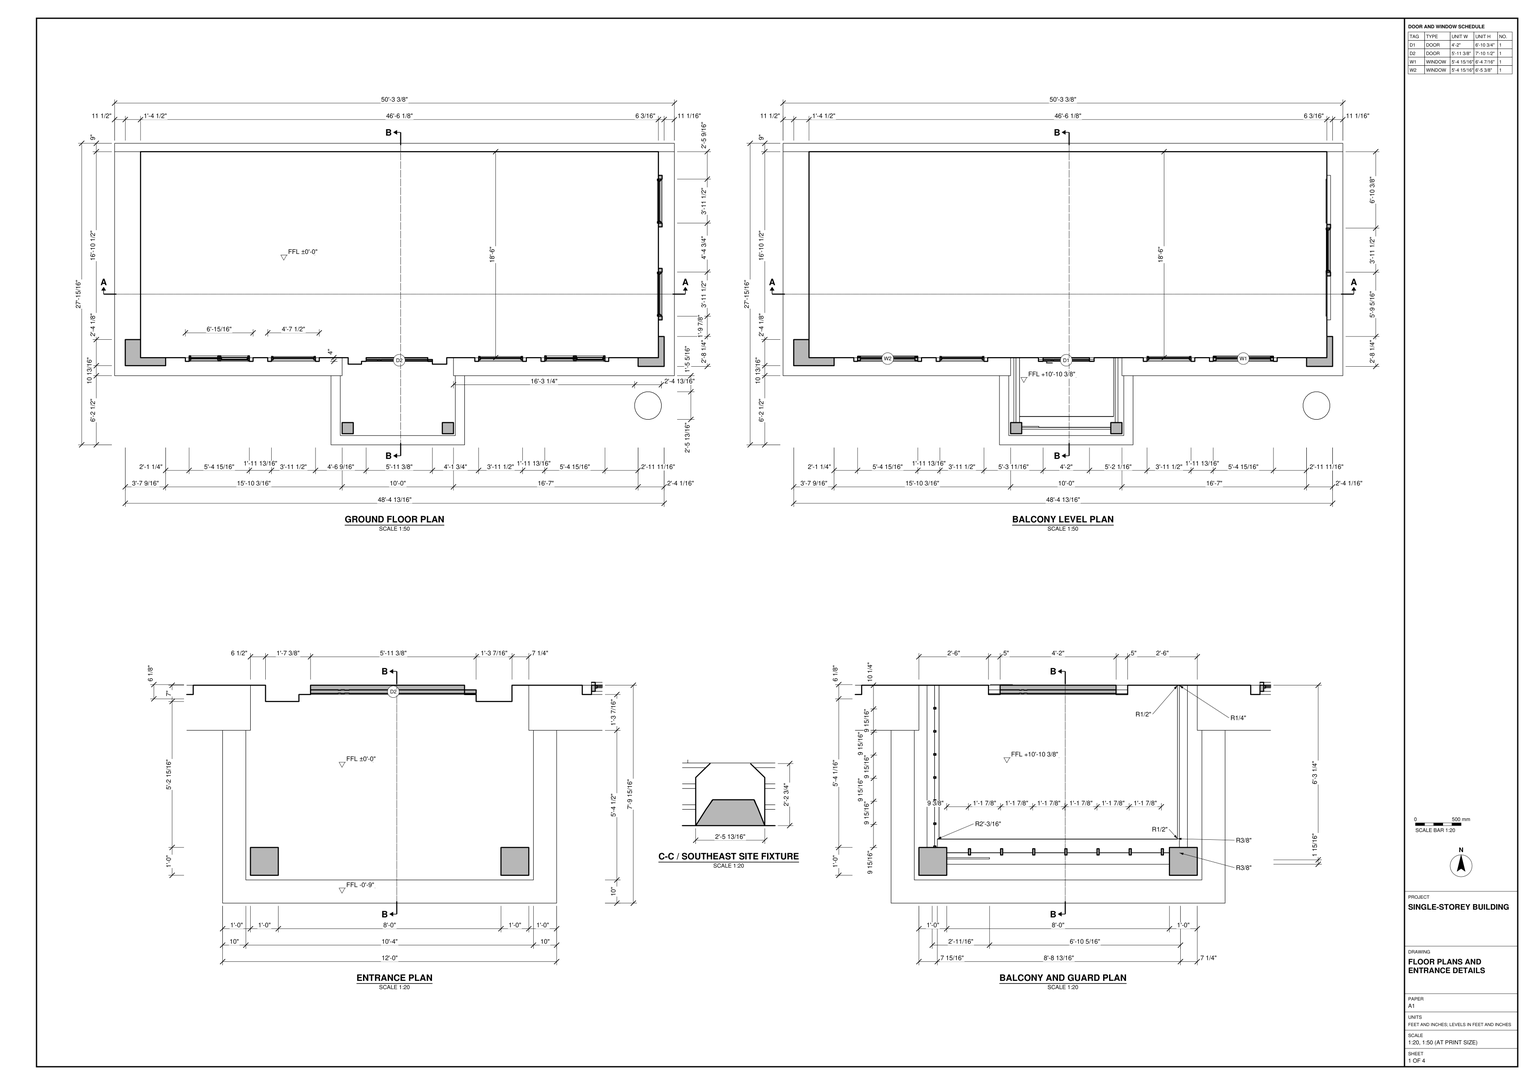
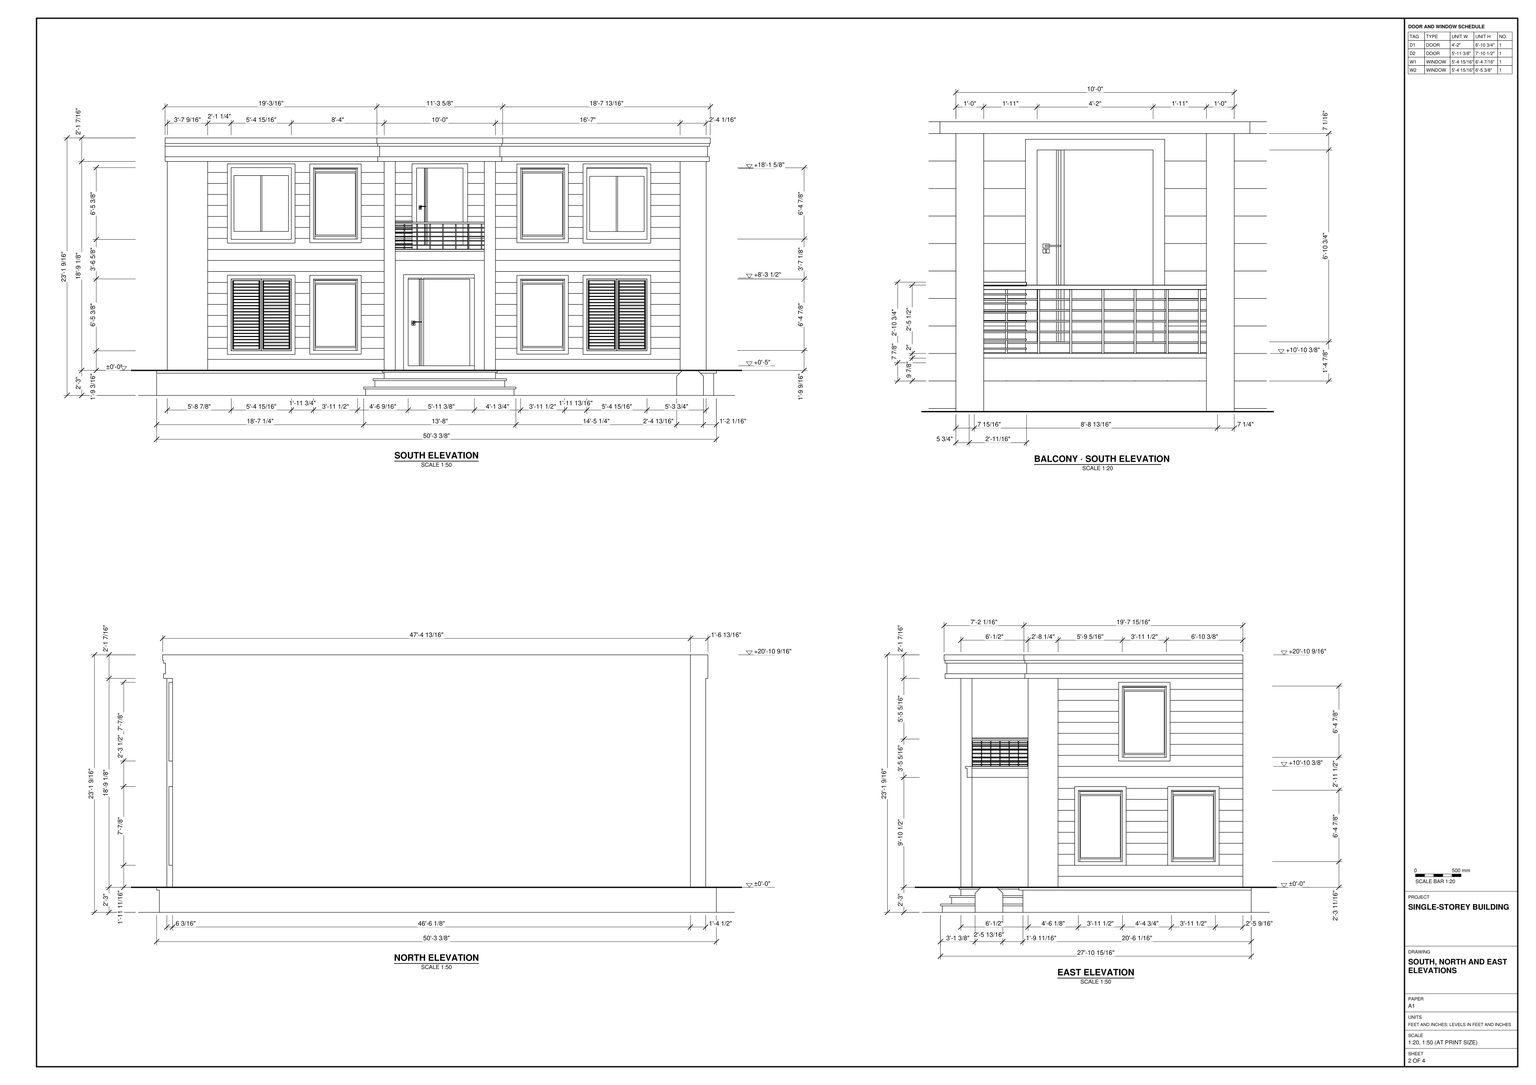
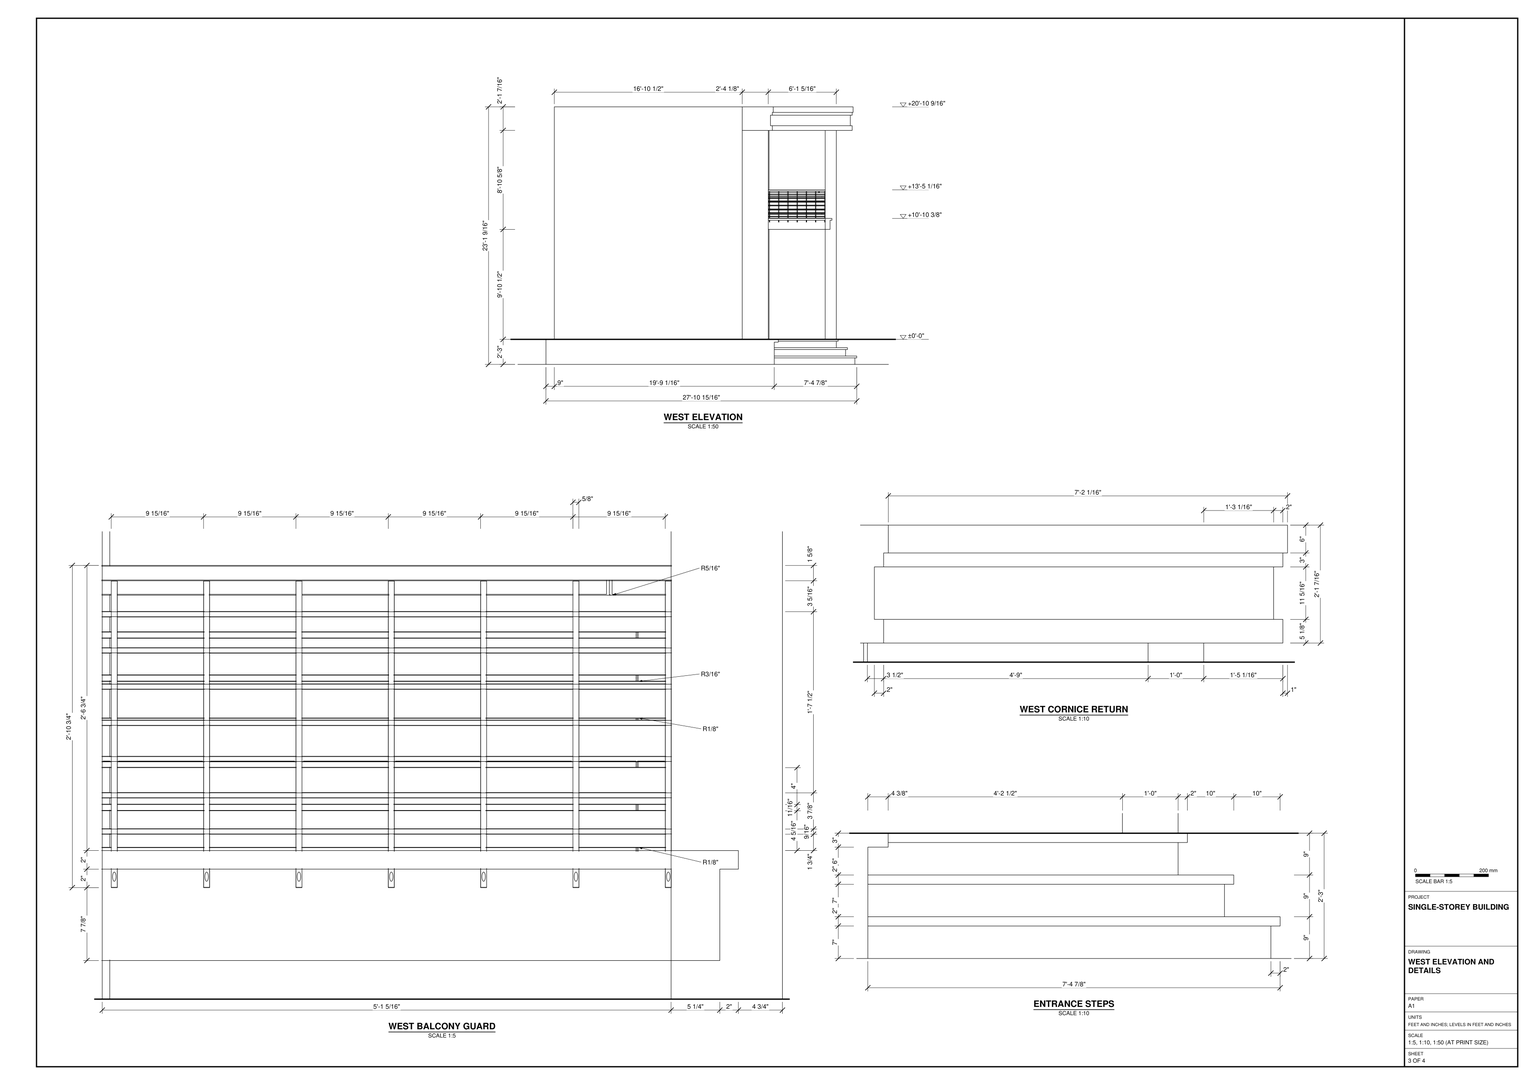
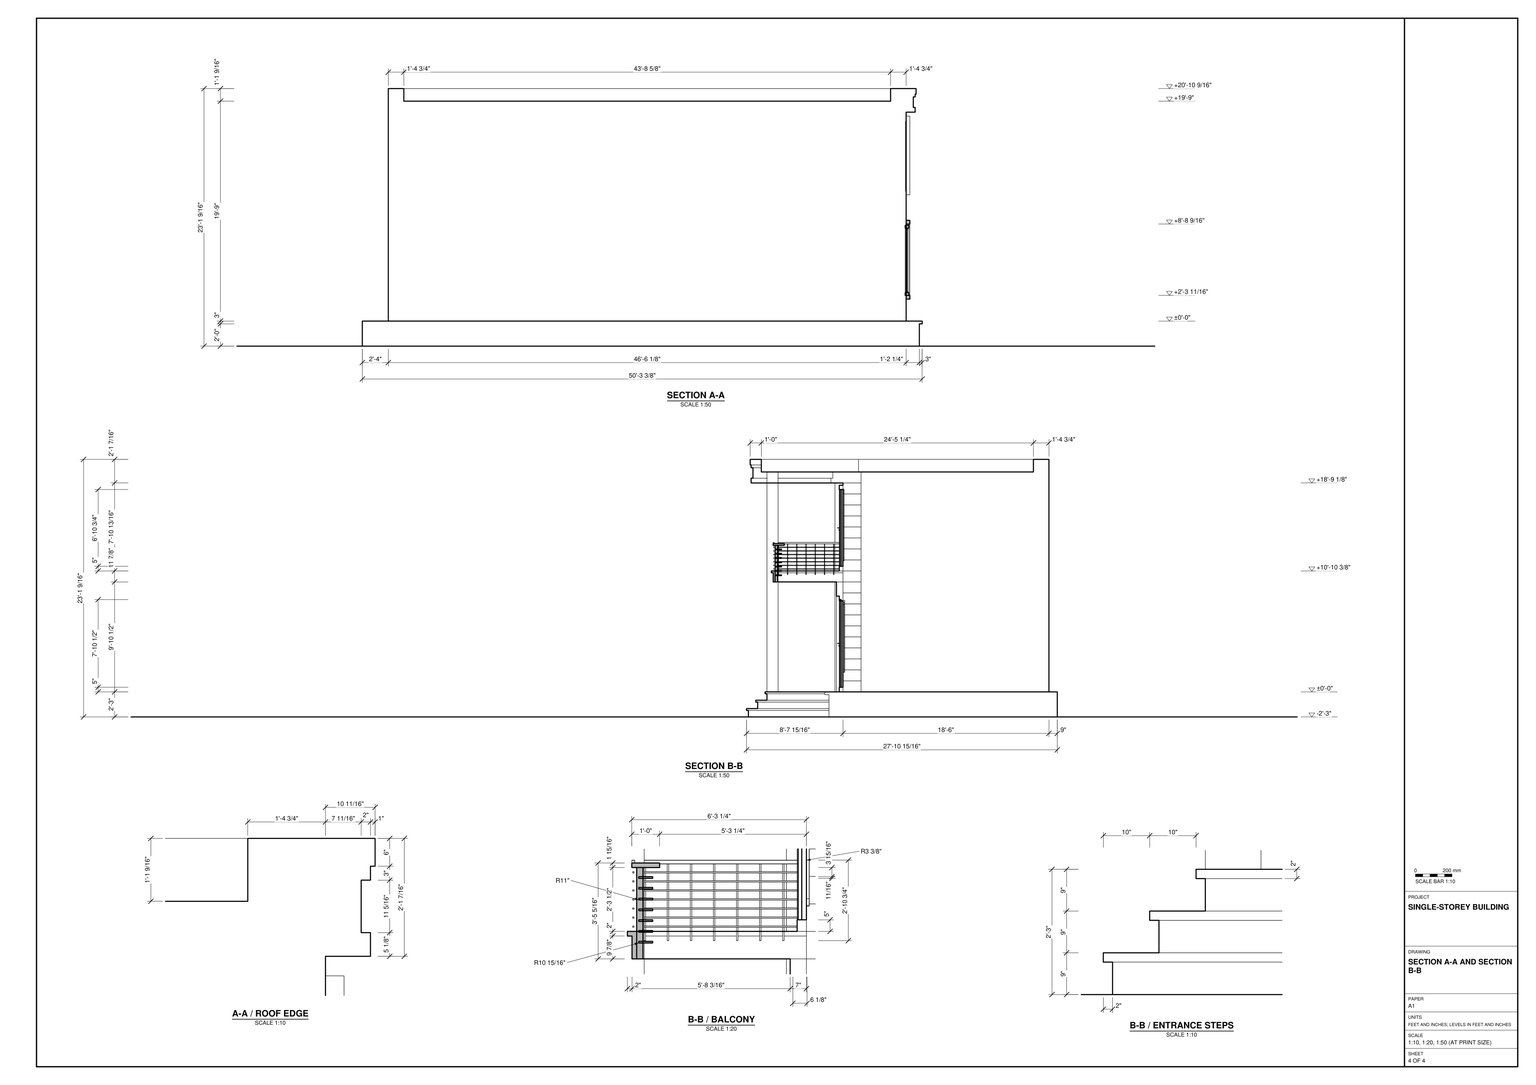
Build the single-storey building and its site in SketchUp using task_files/diagram_01.pdf. Work in feet and inches. The complete model, including the site, measures 82'-5 5/16" along X, 104'-8 7/8" along Y and 23'-1 9/16" along Z. Use ±0'-0" as the ground-floor level. Use the dimensioned plans, rather than the site extents, to set out the building footprint.

Model the floor slab, exterior walls at their drawn thicknesses, and roof with its stepped cornice. On the south face, build the entrance steps and landing beneath the projecting balcony. Align the balcony door over the entrance door, place the square supports at the outer corners, and carry the balcony guard across the front and along the sides. Follow the elevations for the window frames, louvred units and horizontal wall courses, noting how the east window arrangement differs from the south frontage. Include the site fixture shown southeast of the building.

Keep shell elements such as walls, slabs and roof, and any furniture or joinery pieces shown, in separate groups or components. Use components for repeated parts. Decor and loose items may be any suitable library components. Save one SketchUp model as output_files/single_storey_building_with_entrance_steps_and_balcony.skp.

# SketchUp Ruby script. Lengths in inches.
U = 1.inch
M = Sketchup.active_model
def pt(a) = Geom::Point3d.new(a.map { |v| v * U })
def face(e, loops, mat)
  f = e.add_face(loops[0].map { |a| pt(a) })
  loops[1..].each { |l| e.add_face(l.map { |a| pt(a) }).erase! }
  f.material = f.back_material = mat if mat
  f
end
# faces: each face lists its corners as indices into pts; further lists are holes
def faces(e, pts, list, mat = nil) = list.each { |f| face(e, (f[0].is_a?(Array) ? f : [f]).map { |l| l.map { |i| pts[i] } }, mat) }
# xy, xz, yz: faces in a plane at the given z, y or x. An outline is a flat list of corners, or four numbers for a rectangle; further outlines are holes
def ring(l) = l.size == 4 ? [[l[0], l[1]], [l[2], l[1]], [l[2], l[3]], [l[0], l[3]]] : l.each_slice(2).to_a
def flat(e, list, mat, &to3) = list.each { |f| face(e, (f[0].is_a?(Array) ? f : [f]).map { |l| ring(l).map { |u, v| to3.(u, v) } }, mat) }
def xy(e, z, list, mat = nil) = flat(e, list, mat) { |x, y| [x, y, z] }
def xz(e, y, list, mat = nil) = flat(e, list, mat) { |x, z| [x, y, z] }
def yz(e, x, list, mat = nil) = flat(e, list, mat) { |y, z| [x, y, z] }
def lines(e, pts, list) = list.each { |a, b| e.add_line(pt(pts[a]), pt(pts[b])) }
# prism: a flat outline (further loops are holes) pulled along v
def prism(e, loops, v, mat = nil)
  f = face(e, loops, mat); d = Geom::Vector3d.new(v.map { |x| x * U })
  f.pushpull(f.normal.samedirection?(d) ? d.length : -d.length)
end
def box(e, o, s, mat = nil) = prism(e, [[o, [o[0] + s[0], o[1], o[2]], [o[0] + s[0], o[1] + s[1], o[2]], [o[0], o[1] + s[1], o[2]]]], [0, 0, s[2]], mat)
def at(x, y, z, deg = 0) = Geom::Transformation.translation(pt([x, y, z])) * Geom::Transformation.rotation(ORIGIN, Z_AXIS, deg.degrees)
def axes(o, x, y, z) = Geom::Transformation.new([*x, 0, *y, 0, *z, 0, *pt(o).to_a, 1])
def part(name) = M.definitions.add(name)
# library, detail: a bought-in or finely detailed component or shape, given as its bounding box
def library(name, o, s) = part(name).tap { |d| box(d.entities, o, s) }
def detail(e, o, s) = box(e.add_group.entities, o, s)
def put(e, d, t, mat = nil) = e.add_instance(d, t).tap { |i| i.material = mat if mat }
def group(e, t, mat = nil) = e.add_group.tap { |g| g.transformation = t; g.material = mat if mat }.entities
root = M.entities
M.materials.add("GATE RAILINGS").color = [40, 40, 40]
M.materials.add("[0049_Beige]").color = [245, 245, 220]
M.materials.add("[0135_DarkGray]").color = [81, 81, 81]
M.materials.add("[Color_009]").color = [0, 0, 0]
M.materials.add("[Granite Dark Gray]").color = [214, 211, 211]
M.materials.add("[Rough Square Concrete Block]").color = [58, 57, 53]
M.materials.add("[Rough Square Concrete Block]1").color = [53, 52, 49]
M.materials.add("[Translucent_Glass_Gray]").color = [128, 128, 128]
M.materials["[Translucent_Glass_Gray]"].alpha = 0.5
c1 = part("Window+3x7")
g1 = group(c1.entities,at(0,-10,0))
xy(g1,0,[[0,0,36,10]])
xy(g1,4,[[4,0,32,4],[4,4,32,10]],"[Color_009]")
xy(g1,41,[[4,2,32,4],[4,4,32,8]])
xy(g1,43,[[4,2,32,4],[4,4,32,8]],"[Color_009]")
xy(g1,80,[[4,0,32,4],[4,4,32,10]],"[Color_009]")
xy(g1,84,[[0,0,36,10]],"[Color_009]")
xz(g1,0,[[[0,0,36,84],[4,4,32,80]]],"[Color_009]")
xz(g1,2,[[4,41,32,43]],"[Color_009]")
xz(g1,4,[[4,4,32,41],[4,43,32,80]],"[Translucent_Glass_Gray]")
xz(g1,8,[[4,41,32,43]],"[Color_009]")
xz(g1,10,[[[0,0,36,84],[4,4,32,80]]],"[Color_009]")
yz(g1,0,[[0,0,10,84]],"[Color_009]")
yz(g1,4,[[0,4,4,4,4,41,2,41,2,43,4,43,4,80,0,80],[2,41,8,43]])
yz(g1,4,[[4,4,10,4,10,80,4,80,4,43,8,43,8,41,4,41]],"[Color_009]")
yz(g1,32,[[2,41,8,43]])
yz(g1,32,[[0,4,0,80,4,80,4,43,2,43,2,41,4,41,4,4],[4,4,4,41,8,41,8,43,4,43,4,80,10,80,10,4]],"[Color_009]")
yz(g1,36,[[0,0,10,84]],"[Color_009]")
c2 = library("JSilva Jalousie",[-31.89,-0.05,0.1],[63.78,4.97,70.86])
c3 = library("Window assembly",[84,-6,0],[60,6,73.01])
c4 = library("Horizontal railing bar",[-171.26,0.98,-0.71],[237.2,23.72,0.71])
c5 = library("Railing post",[0,-1.77,-6.85],[2.07,1.28,39.37])
c6 = library("Group\#5",[-171.26,0,0],[238.19,24.7,1.97])
c7 = part("Balcony railing")
put(c7.entities,c4,at(44.24,-0.6875,35.43),"GATE RAILINGS")
put(c7.entities,c4,at(44.24,-0.6875,30.79),"GATE RAILINGS")
put(c7.entities,c4,at(44.24,-0.6875,26.14),"GATE RAILINGS")
put(c7.entities,c4,at(44.24,-0.6875,21.5),"GATE RAILINGS")
put(c7.entities,c4,at(44.24,-0.6875,16.85),"GATE RAILINGS")
put(c7.entities,c4,at(44.24,-0.6875,12.2),"GATE RAILINGS")
put(c7.entities,c4,at(44.24,-0.6875,7.56),"GATE RAILINGS")
put(c7.entities,c5,at(60.92,1.38,6.85))
put(c7.entities,c5,at(92.41,1.38,6.85))
put(c7.entities,c5,at(29.42,1.38,6.85))
put(c7.entities,c5,at(-2.07,1.38,6.85))
put(c7.entities,c5,at(-33.57,1.38,6.85))
put(c7.entities,c5,at(-65.07,1.38,6.85))
put(c7.entities,c5,at(-96.5625,1.38,6.85))
put(c7.entities,c6,at(44.24,-0.6875,39.37),"GATE RAILINGS")
c8 = library("PUERTA",[0,-2.28,0],[35.43,6.14,94.49])
c9 = library("POTTED+PLANT+FERN",[-10.17,-13.1,0],[24.03,24.03,12.74])
xy(root,0,[[135.18,752.25,735.55,998.32]],"[0049_Beige]")
xy(root,0,[[[0,0,989.3125,1256.875],[360.43,665.38,520.43,752.25]],[360.43,665.38,520.43,752.25]],"[Granite Dark Gray]")
xy(root,7,[[358.43,663.38,360.43,752.25],[360.43,663.38,522.43,665.38],[520.43,665.38,522.43,752.25]],"[Granite Dark Gray]")
xy(root,9,[[358.43,663.38,522.43,663.38,522.43,752.25,510.43,752.25,510.43,675.38,370.43,675.38,370.43,752.25,358.43,752.25]],"[Granite Dark Gray]")
xy(root,16,[[368.43,673.38,370.43,752.25],[370.43,673.38,512.43,675.38],[510.43,675.38,512.43,752.25]],"[Granite Dark Gray]")
xy(root,18,[[368.43,673.38,512.43,673.38,512.43,752.25,500.43,752.25,500.43,685.38,380.43,685.38,380.43,752.25,368.43,752.25]],"[Granite Dark Gray]")
xy(root,24,[[135.18,747.88,380.43,752.25],[500.43,747.88,500.43,752.25,735.55,752.25,735.55,758.32,738.55,758.32,738.55,747.88],[735.55,758.32,738.55,998.32]],"[0049_Beige]")
xy(root,25,[[378.43,683.38,392.43,685.38],[392.43,683.38,502.43,685.38],[378.43,685.38,380.43,747.88],[500.43,685.38,502.43,747.88]],"[Granite Dark Gray]")
xy(root,27,[[380.43,685.38,392.43,697.38],[488.43,685.38,500.43,697.38],[386.93,760.32,401.32,760.32,401.32,763.32,477.72,763.32,477.72,760.32,493.18,760.32,493.18,767.32,721.3,767.32,721.3,989.32,163.18,989.32,163.18,767.32,386.93,767.32]])
xy(root,27,[[135.18,747.88,380.43,747.88,380.43,767.32,190.21,767.32,190.21,758.69,146.68,758.69,146.68,786.8,163.18,786.8,163.18,989.32,135.18,989.32],[500.43,747.88,738.55,747.88,738.55,989.32,721.3,989.32,721.3,790.13,727.5,790.13,727.5,757.88,699.43,757.88,699.43,767.32,500.43,767.32],[135.18,989.32,738.55,998.32]],"[0049_Beige]")
xy(root,27,[[[378.43,683.38,502.43,683.38,502.43,747.88,500.43,747.88,500.43,767.32,493.18,767.32,493.18,760.32,477.72,760.32,477.72,763.32,401.32,763.32,401.32,760.32,386.93,760.32,386.93,767.32,380.43,767.32,380.43,747.88,378.43,747.88],[488.43,685.38,500.43,697.38],[380.43,685.38,392.43,697.38]]],"[Granite Dark Gray]")
xy(root,32,[[406.32,763.32,472.72,767.32]],"[0135_DarkGray]")
xy(root,44.17,[[211.47,763.32,284.41,767.32],[594.81,763.32,667.74,767.32]],"[0049_Beige]")
xy(root,44.55,[[300.24,763.32,355.74,767.32],[523.47,763.32,578.97,767.32]],"[0049_Beige]")
xy(root,48.17,[[215.47,763.32,280.41,767.32],[598.81,763.32,663.74,767.32]],"[0049_Beige]")
xy(root,48.55,[[304.24,763.32,351.74,767.32],[527.47,763.32,574.97,767.32]],"[0049_Beige]")
xy(root,50.7,[[721.3,808.03,725.3,863.53],[721.3,908.28,725.3,963.78]],"[0049_Beige]")
xy(root,54.7,[[721.3,812.03,725.3,859.53],[721.3,912.28,725.3,959.78]],"[0049_Beige]")
xy(root,125.2,[[406.32,763.32,472.72,767.32]],"[0135_DarkGray]")
xy(root,125.41,[[304.24,763.32,351.74,767.32],[527.47,763.32,574.97,767.32]],"[0049_Beige]")
xy(root,125.55,[[215.47,763.32,280.41,767.32],[598.81,763.32,663.74,767.32]],"[0049_Beige]")
xy(root,129.41,[[300.24,763.32,355.74,767.32],[523.47,763.32,578.97,767.32]],"[0049_Beige]")
xy(root,129.55,[[211.47,763.32,284.41,767.32],[594.81,763.32,667.74,767.32]],"[0049_Beige]")
xy(root,130.2,[[401.32,760.32,477.72,763.32]],"[Rough Square Concrete Block]1")
xy(root,131.56,[[721.3,812.03,725.3,859.53],[721.3,912.28,725.3,959.78]],"[0049_Beige]")
xy(root,135.56,[[721.3,808.03,725.3,863.53],[721.3,908.28,725.3,963.78]],"[0049_Beige]")
xy(root,145.5,[[380.43,692.13,380.43,697.38,386.93,697.38,386.93,760.32,493.18,760.32,493.18,697.38,500.43,697.38,500.43,692.13]],"[Rough Square Concrete Block]")
xy(root,155.35,[[380.43,690.13,500.43,692.13],[383.93,697.38,386.93,767.32],[493.18,697.38,496.18,767.32]],"[Granite Dark Gray]")
xy(root,157.35,[[380.43,690.13,500.43,690.13,500.43,697.38,496.18,697.38,496.18,767.32,470.43,767.32,470.43,763.32,410.43,763.32,410.43,767.32,383.93,767.32,383.93,697.38,380.43,697.38]],"[Granite Dark Gray]")
xy(root,162.35,[[415.43,763.32,465.43,767.32]],"[0049_Beige]")
xy(root,163.08,[[721.3,855.41,725.3,910.91]],"[0049_Beige]")
xy(root,164.17,[[211.47,763.32,284.41,767.32],[594.81,763.32,667.74,767.32]],"[0049_Beige]")
xy(root,164.55,[[300.24,763.32,355.74,767.32],[523.47,763.32,578.97,767.32]],"[0049_Beige]")
xy(root,167.08,[[721.3,859.41,725.3,906.91]],"[0049_Beige]")
xy(root,168.17,[[215.47,763.32,280.41,767.32],[598.81,763.32,663.74,767.32]],"[0049_Beige]")
xy(root,168.55,[[304.24,763.32,351.74,767.32],[527.47,763.32,574.97,767.32]],"[0049_Beige]")
xy(root,243.94,[[721.3,859.41,725.3,906.91]],"[0049_Beige]")
xy(root,245.08,[[415.43,763.32,465.43,767.32]],"[0049_Beige]")
xy(root,245.41,[[304.24,763.32,351.74,767.32],[527.47,763.32,574.97,767.32]],"[0049_Beige]")
xy(root,245.55,[[215.47,763.32,280.41,767.32],[598.81,763.32,663.74,767.32]],"[0049_Beige]")
xy(root,247.94,[[721.3,855.41,725.3,910.91]],"[0049_Beige]")
xy(root,249.41,[[300.24,763.32,355.74,767.32],[523.47,763.32,578.97,767.32]],"[0049_Beige]")
xy(root,249.55,[[211.47,763.32,284.41,767.32],[594.81,763.32,667.74,767.32]],"[0049_Beige]")
xy(root,249.68,[[410.43,763.32,470.43,767.32]],"[0049_Beige]")
xy(root,252.15,[[699.43,757.88,699.43,767.32,721.3,767.32,721.3,790.13,727.5,790.13,727.5,757.88]])
xy(root,252.15,[[373.55,668.32,507.18,754.38],[144.37,754.38,144.37,786.8,146.68,786.8,146.68,758.69,190.21,758.69,190.21,767.32,699.43,767.32,699.43,754.38],[699.43,754.38,731,757.88],[727.5,757.88,731,790.13],[721.3,790.13,731,989.32]],"[0049_Beige]")
xy(root,257.25,[[373.55,668.32,505.18,670.32],[505.18,668.32,507.18,754.38],[373.55,670.32,375.55,756.38],[144.37,754.38,373.55,756.38],[505.18,754.38,729,756.38],
  [729,754.38,731,989.32]],"[0049_Beige]")
xy(root,264,[[384.55,679.32,496.18,679.32,496.18,685.38,488.43,685.38,488.43,697.38,496.18,697.38,496.18,784.07,704.55,784.07,704.55,972.57,179.93,972.57,179.93,784.07,384.55,784.07,384.55,697.38,392.43,697.38,392.43,685.38,384.55,685.38],[384.55,685.38,392.43,697.38],[488.43,685.38,496.18,697.38]],"[0049_Beige]")
xy(root,268.5625,[[373.55,668.32,505.18,670.32],[505.18,668.32,507.18,754.38],[373.55,670.32,375.55,756.38],[144.37,754.38,373.55,756.38],[505.18,754.38,731,756.38],
  [729,756.38,731,989.32]],"[0049_Beige]")
xy(root,271.5625,[[372.55,667.32,372.55,670.32,373.55,670.32,373.55,668.32,505.18,668.32,505.18,667.32],[505.18,667.32,505.18,668.32,507.18,668.32,507.18,753.38,508.18,753.38,508.18,667.32],[372.55,670.32,373.55,754.38],[144.37,753.38,372.55,754.38],[507.18,753.38,507.18,754.38,731,754.38,731,756.38,732,756.38,732,753.38],
  [731,756.38,732,989.32]],"[0135_DarkGray]")
xy(root,277.5625,[[[372.55,667.32,508.18,667.32,508.18,753.38,732,753.38,732,989.32,163.18,989.32,163.18,786.8,144.37,786.8,144.37,753.38,372.55,753.38],[384.55,679.32,384.55,784.07,179.93,784.07,179.93,972.57,704.55,972.57,704.55,784.07,496.18,784.07,496.18,679.32]]],"[0135_DarkGray]")
xz(root,663.38,[[358.43,7,522.43,9]],"[Granite Dark Gray]")
xz(root,665.38,[[360.43,0,520.43,7]],"[Granite Dark Gray]")
xz(root,667.32,[[372.55,271.5625,508.18,277.5625]],"[0135_DarkGray]")
xz(root,668.32,[[373.55,252.15,507.18,257.25],[373.55,268.5625,507.18,271.5625]],"[0049_Beige]")
xz(root,670.32,[[375.55,257.25,505.18,268.5625]],"[0049_Beige]")
xz(root,673.38,[[368.43,16,512.43,18]],"[Granite Dark Gray]")
xz(root,675.38,[[370.43,9,510.43,16]],"[Granite Dark Gray]")
xz(root,679.32,[[384.55,264,496.18,277.5625]],"[0049_Beige]")
xz(root,683.38,[[378.43,25,502.43,27]],"[Granite Dark Gray]")
xz(root,685.38,[[380.43,18,500.43,25]],"[Granite Dark Gray]")
xz(root,685.38,[[380.43,27,392.43,264],[488.43,27,500.43,264]],"[Rough Square Concrete Block]")
xz(root,690.13,[[380.43,155.35,500.43,157.35]],"[Granite Dark Gray]")
xz(root,692.13,[[380.43,145.5,500.43,155.35]],"[Rough Square Concrete Block]")
xz(root,697.38,[[380.43,145.5,386.93,155.35],[493.18,145.5,493.18,155.35,496.18,155.35,496.18,157.35,500.43,157.35,500.43,145.5],[380.43,155.35,383.93,157.35]])
xz(root,697.38,[[380.43,27,380.43,145.5,386.93,145.5,386.93,155.35,383.93,155.35,383.93,157.35,380.43,157.35,380.43,264,392.43,264,392.43,27],[488.43,27,488.43,264,500.43,264,500.43,157.35,496.18,157.35,496.18,155.35,493.18,155.35,493.18,145.5,500.43,145.5,500.43,27]],"[Rough Square Concrete Block]")
xz(root,747.88,[[135.18,24,380.43,24,380.43,25,378.43,25,378.43,27,135.18,27],[500.43,24,738.55,24,738.55,27,502.43,27,502.43,25,500.43,25]],"[0049_Beige]")
xz(root,752.25,[[135.18,0,360.43,0,360.43,7,358.43,7,358.43,9,370.43,9,370.43,16,368.43,16,368.43,18,380.43,18,380.43,24,135.18,24],[520.43,0,735.55,0,735.55,24,500.43,24,500.43,18,512.43,18,512.43,16,510.43,16,510.43,9,522.43,9,522.43,7,520.43,7]],"[0049_Beige]")
xz(root,753.38,[[144.37,271.5625,372.55,277.5625],[508.18,271.5625,732,277.5625]],"[0135_DarkGray]")
xz(root,754.38,[[144.37,252.15,373.55,257.25],[507.18,252.15,731,257.25],[144.37,268.5625,373.55,271.5625],[507.18,268.5625,731,271.5625]],"[0049_Beige]")
xz(root,756.38,[[144.37,257.25,375.55,268.5625],[505.18,257.25,729,268.5625]],"[0049_Beige]")
xz(root,757.88,[[699.43,27,727.5,252.15]],"[Rough Square Concrete Block]")
xz(root,758.69,[[146.68,27,190.21,252.15]],"[Rough Square Concrete Block]")
xz(root,760.32,[[386.93,27,401.32,27,401.32,130.2,477.72,130.2,477.72,27,493.18,27,493.18,145.5,386.93,145.5]],"[Rough Square Concrete Block]1")
xz(root,763.32,[[[211.47,44.17,284.41,129.55],[215.47,48.17,280.41,125.55]],[[594.81,44.17,667.74,129.55],[598.81,48.17,663.74,125.55]],[[300.24,44.55,355.74,129.41],[304.24,48.55,351.74,125.41]],[[523.47,44.55,578.97,129.41],[527.47,48.55,574.97,125.41]],[[410.43,157.35,470.43,249.68],[415.43,162.35,465.43,245.08]],
  [[211.47,164.17,284.41,249.55],[215.47,168.17,280.41,245.55]],[[594.81,164.17,667.74,249.55],[598.81,168.17,663.74,245.55]],[[300.24,164.55,355.74,249.41],[304.24,168.55,351.74,245.41]],[[523.47,164.55,578.97,249.41],[527.47,168.55,574.97,245.41]]],"[0049_Beige]")
xz(root,763.32,[[[401.32,27,477.72,130.2],[406.32,32,472.72,125.2]]],"[0135_DarkGray]")
xz(root,767.32,[[163.18,27,190.21,38.85],[699.43,27,721.3,38.85],[163.18,38.85,190.21,50.7],[699.43,38.85,721.3,50.7],[163.18,50.7,190.21,62.55],
  [699.43,50.7,721.3,62.55],[163.18,62.55,190.21,74.4],[699.43,62.55,721.3,74.4],[163.18,74.4,190.21,86.25],[699.43,74.4,721.3,86.25],
  [163.18,86.25,190.21,98.1],[699.43,86.25,721.3,98.1],[163.18,98.1,190.21,109.95],[699.43,98.1,721.3,109.95],[163.18,109.95,190.21,121.8],
  [699.43,109.95,721.3,121.8],[163.18,121.8,190.21,133.65],[699.43,121.8,721.3,133.65],[163.18,133.65,190.21,145.5],[699.43,133.65,721.3,145.5],
  [163.18,145.5,190.21,157.35],[699.43,145.5,721.3,157.35],[163.18,157.35,190.21,169.2],[699.43,157.35,721.3,169.2],[215.47,168.17,280.41,169.2],
  [598.81,168.17,663.74,169.2],[304.24,168.55,351.74,169.2],[527.47,168.55,574.97,169.2],[163.18,169.2,190.21,181.05],[699.43,169.2,721.3,181.05],
  [163.18,181.05,190.21,192.9],[699.43,181.05,721.3,192.9],[163.18,192.9,190.21,204.75],[699.43,192.9,721.3,204.75],[163.18,204.75,190.21,216.6],
  [699.43,204.75,721.3,216.6],[163.18,216.6,190.21,228.45],[699.43,216.6,721.3,228.45],[163.18,228.45,190.21,240.3],[699.43,228.45,721.3,240.3],
  [163.18,240.3,190.21,252.15],[699.43,240.3,721.3,252.15]])
xz(root,767.32,[[190.21,27,386.93,38.85],[493.18,27,699.43,38.85],[190.21,38.85,386.93,38.85,386.93,50.7,355.74,50.7,355.74,44.55,300.24,44.55,300.24,50.7,284.41,50.7,284.41,44.17,211.47,44.17,211.47,50.7,190.21,50.7],[493.18,38.85,699.43,38.85,699.43,50.7,667.74,50.7,667.74,44.17,594.81,44.17,594.81,50.7,578.97,50.7,578.97,44.55,523.47,44.55,523.47,50.7,493.18,50.7],[190.21,50.7,211.47,62.55],
  [284.41,50.7,300.24,62.55],[355.74,50.7,386.93,62.55],[493.18,50.7,523.47,62.55],[578.97,50.7,594.81,62.55],[667.74,50.7,699.43,62.55],
  [190.21,62.55,211.47,74.4],[284.41,62.55,300.24,74.4],[355.74,62.55,386.93,74.4],[493.18,62.55,523.47,74.4],[578.97,62.55,594.81,74.4],
  [667.74,62.55,699.43,74.4],[190.21,74.4,211.47,86.25],[284.41,74.4,300.24,86.25],[355.74,74.4,386.93,86.25],[493.18,74.4,523.47,86.25],
  [578.97,74.4,594.81,86.25],[667.74,74.4,699.43,86.25],[190.21,86.25,211.47,98.1],[284.41,86.25,300.24,98.1],[355.74,86.25,386.93,98.1],
  [493.18,86.25,523.47,98.1],[578.97,86.25,594.81,98.1],[667.74,86.25,699.43,98.1],[190.21,98.1,211.47,109.95],[284.41,98.1,300.24,109.95],
  [355.74,98.1,386.93,109.95],[493.18,98.1,523.47,109.95],[578.97,98.1,594.81,109.95],[667.74,98.1,699.43,109.95],[190.21,109.95,211.47,121.8],
  [284.41,109.95,300.24,121.8],[355.74,109.95,386.93,121.8],[493.18,109.95,523.47,121.8],[578.97,109.95,594.81,121.8],[667.74,109.95,699.43,121.8],
  [190.21,121.8,211.47,121.8,211.47,129.55,284.41,129.55,284.41,121.8,300.24,121.8,300.24,129.41,355.74,129.41,355.74,121.8,386.93,121.8,386.93,133.65,190.21,133.65],[493.18,121.8,523.47,121.8,523.47,129.41,578.97,129.41,578.97,121.8,594.81,121.8,594.81,129.55,667.74,129.55,667.74,121.8,699.43,121.8,699.43,133.65,493.18,133.65],[190.21,133.65,386.93,145.5],[493.18,133.65,699.43,145.5],[190.21,145.5,386.93,145.5,386.93,155.35,383.93,155.35,383.93,157.35,190.21,157.35],
  [493.18,145.5,699.43,145.5,699.43,157.35,496.18,157.35,496.18,155.35,493.18,155.35],[190.21,157.35,410.43,157.35,410.43,169.2,355.74,169.2,355.74,164.55,300.24,164.55,300.24,169.2,284.41,169.2,284.41,164.17,211.47,164.17,211.47,169.2,190.21,169.2],[470.43,157.35,699.43,157.35,699.43,169.2,667.74,169.2,667.74,164.17,594.81,164.17,594.81,169.2,578.97,169.2,578.97,164.55,523.47,164.55,523.47,169.2,470.43,169.2],[190.21,169.2,211.47,181.05],[284.41,169.2,300.24,181.05],
  [355.74,169.2,410.43,181.05],[470.43,169.2,523.47,181.05],[578.97,169.2,594.81,181.05],[667.74,169.2,699.43,181.05],[190.21,181.05,211.47,192.9],
  [284.41,181.05,300.24,192.9],[355.74,181.05,410.43,192.9],[470.43,181.05,523.47,192.9],[578.97,181.05,594.81,192.9],[667.74,181.05,699.43,192.9],
  [190.21,192.9,211.47,204.75],[284.41,192.9,300.24,204.75],[355.74,192.9,410.43,204.75],[470.43,192.9,523.47,204.75],[578.97,192.9,594.81,204.75],
  [667.74,192.9,699.43,204.75],[190.21,204.75,211.47,216.6],[284.41,204.75,300.24,216.6],[355.74,204.75,410.43,216.6],[470.43,204.75,523.47,216.6],
  [578.97,204.75,594.81,216.6],[667.74,204.75,699.43,216.6],[190.21,216.6,211.47,228.45],[284.41,216.6,300.24,228.45],[355.74,216.6,410.43,228.45],
  [470.43,216.6,523.47,228.45],[578.97,216.6,594.81,228.45],[667.74,216.6,699.43,228.45],[190.21,228.45,211.47,240.3],[284.41,228.45,300.24,240.3],
  [355.74,228.45,410.43,240.3],[470.43,228.45,523.47,240.3],[578.97,228.45,594.81,240.3],[667.74,228.45,699.43,240.3],[190.21,240.3,211.47,240.3,211.47,249.55,284.41,249.55,284.41,240.3,300.24,240.3,300.24,249.41,355.74,249.41,355.74,240.3,410.43,240.3,410.43,249.68,470.43,249.68,470.43,240.3,523.47,240.3,523.47,249.41,578.97,249.41,578.97,240.3,594.81,240.3,594.81,249.55,667.74,249.55,667.74,240.3,699.43,240.3,699.43,252.15,190.21,252.15]],"[0049_Beige]")
xz(root,767.32,[[406.32,32,472.72,125.2],[215.47,48.17,280.41,125.55],[598.81,48.17,663.74,125.55],[304.24,48.55,351.74,125.41],[527.47,48.55,574.97,125.41],
  [415.43,162.35,465.43,245.08],[215.47,169.2,280.41,245.55],[304.24,169.2,351.74,245.41],[527.47,169.2,574.97,245.41],[598.81,169.2,663.74,245.55]],"[0135_DarkGray]")
xz(root,784.07,[[179.93,264,380.43,277.5625],[380.43,264,384.55,277.5625],[496.18,264,500.43,277.5625],[500.43,264,704.55,277.5625]],"[0049_Beige]")
xz(root,786.8,[[146.68,27,146.68,252.15,144.37,252.15,144.37,277.5625,163.18,277.5625,163.18,27]],"[0049_Beige]")
xz(root,790.13,[[721.3,27,727.5,252.15]],"[Rough Square Concrete Block]")
xz(root,808.03,[[721.3,50.7,725.3,135.56]],"[0049_Beige]")
xz(root,812.03,[[721.3,54.7,725.3,131.56]],"[0049_Beige]")
xz(root,855.41,[[721.3,163.08,725.3,247.94]],"[0049_Beige]")
xz(root,859.41,[[721.3,167.08,725.3,243.94]],"[0049_Beige]")
xz(root,859.53,[[721.3,54.7,725.3,131.56]],"[0049_Beige]")
xz(root,863.53,[[721.3,50.7,725.3,135.56]],"[0049_Beige]")
xz(root,906.91,[[721.3,167.08,725.3,243.94]],"[0049_Beige]")
xz(root,908.28,[[721.3,50.7,725.3,135.56]],"[0049_Beige]")
xz(root,910.91,[[721.3,163.08,725.3,247.94]],"[0049_Beige]")
xz(root,912.28,[[721.3,54.7,725.3,131.56]],"[0049_Beige]")
xz(root,959.78,[[721.3,54.7,725.3,131.56]],"[0049_Beige]")
xz(root,963.78,[[721.3,50.7,725.3,135.56]],"[0049_Beige]")
xz(root,972.57,[[179.93,264,704.55,277.5625]],"[0049_Beige]")
xz(root,989.32,[[163.18,27,163.18,277.5625,732,277.5625,732,271.5625,731,271.5625,731,268.5625,729,268.5625,729,257.25,731,257.25,731,252.15,721.3,252.15,721.3,27]],"[0049_Beige]")
xz(root,998.32,[[135.18,0,135.18,27,738.55,27,738.55,24,735.55,24,735.55,0]],"[0049_Beige]")
yz(root,135.18,[[752.25,0,752.25,24,747.88,24,747.88,27,998.32,27,998.32,0]],"[0049_Beige]")
yz(root,144.37,[[754.38,252.15,754.38,257.25,756.38,257.25,756.38,268.5625,754.38,268.5625,754.38,271.5625,753.38,271.5625,753.38,277.5625,786.8,277.5625,786.8,252.15]],"[0049_Beige]")
yz(root,146.68,[[758.69,27,786.8,252.15]],"[Rough Square Concrete Block]")
yz(root,163.18,[[767.32,27,786.8,38.85],[767.32,38.85,786.8,50.7],[767.32,50.7,786.8,62.55],[767.32,62.55,786.8,74.4],[767.32,74.4,786.8,86.25],
  [767.32,86.25,786.8,98.1],[767.32,98.1,786.8,109.95],[767.32,109.95,786.8,121.8],[767.32,121.8,786.8,133.65],[767.32,133.65,786.8,145.5],
  [767.32,145.5,786.8,157.35],[767.32,157.35,786.8,169.2],[767.32,169.2,786.8,181.05],[767.32,181.05,786.8,192.9],[767.32,192.9,786.8,204.75],
  [767.32,204.75,786.8,216.6],[767.32,216.6,786.8,228.45],[767.32,228.45,786.8,240.3],[767.32,240.3,786.8,252.15]])
yz(root,163.18,[[786.8,27,989.32,277.5625]],"[0049_Beige]")
yz(root,179.93,[[784.07,264,972.57,277.5625]],"[0049_Beige]")
yz(root,190.21,[[758.69,27,767.32,252.15]],"[Rough Square Concrete Block]")
yz(root,211.47,[[763.32,44.17,767.32,129.55],[763.32,164.17,767.32,249.55]],"[0049_Beige]")
yz(root,215.47,[[763.32,48.17,767.32,125.55],[763.32,168.17,767.32,245.55]],"[0049_Beige]")
yz(root,280.41,[[763.32,48.17,767.32,125.55],[763.32,168.17,767.32,245.55]],"[0049_Beige]")
yz(root,284.41,[[763.32,44.17,767.32,129.55],[763.32,164.17,767.32,249.55]],"[0049_Beige]")
yz(root,300.24,[[763.32,44.55,767.32,129.41],[763.32,164.55,767.32,249.41]],"[0049_Beige]")
yz(root,304.24,[[763.32,48.55,767.32,125.41],[763.32,168.55,767.32,245.41]],"[0049_Beige]")
yz(root,351.74,[[763.32,48.55,767.32,125.41],[763.32,168.55,767.32,245.41]],"[0049_Beige]")
yz(root,355.74,[[763.32,44.55,767.32,129.41],[763.32,164.55,767.32,249.41]],"[0049_Beige]")
yz(root,358.43,[[663.38,7,752.25,9]],"[Granite Dark Gray]")
yz(root,360.43,[[665.38,0,752.25,7]],"[Granite Dark Gray]")
yz(root,368.43,[[673.38,16,752.25,18]],"[Granite Dark Gray]")
yz(root,370.43,[[675.38,9,752.25,16]],"[Granite Dark Gray]")
yz(root,372.55,[[667.32,271.5625,753.38,277.5625]],"[0135_DarkGray]")
yz(root,373.55,[[668.32,252.15,754.38,257.25],[668.32,268.5625,754.38,271.5625]],"[0049_Beige]")
yz(root,375.55,[[670.32,257.25,756.38,268.5625]],"[0049_Beige]")
yz(root,378.43,[[683.38,25,747.88,27]],"[Granite Dark Gray]")
yz(root,380.43,[[685.38,18,685.38,25,747.88,25,747.88,24,752.25,24,752.25,18]],"[Granite Dark Gray]")
yz(root,380.43,[[685.38,27,685.38,252.15,697.38,252.15,697.38,157.35,690.13,157.35,690.13,155.35,692.13,155.35,692.13,145.5,697.38,145.5,697.38,27],[692.13,145.5,692.13,155.35,690.13,155.35,690.13,157.35,697.38,157.35,697.38,145.5]],"[Rough Square Concrete Block]")
yz(root,383.93,[[697.38,155.35,767.32,157.35]],"[Granite Dark Gray]")
yz(root,384.55,[[679.32,264,784.07,277.5625]],"[0049_Beige]")
yz(root,386.93,[[697.38,145.5,767.32,155.35]],"[Rough Square Concrete Block]")
yz(root,386.93,[[760.32,27,767.32,145.5]],"[Rough Square Concrete Block]1")
yz(root,392.43,[[685.38,27,697.38,264]],"[Rough Square Concrete Block]")
yz(root,401.32,[[760.32,27,763.32,130.2]],"[Rough Square Concrete Block]1")
yz(root,406.32,[[763.32,32,767.32,125.2]],"[0135_DarkGray]")
yz(root,410.43,[[763.32,157.35,767.32,249.68]],"[0049_Beige]")
yz(root,415.43,[[763.32,162.35,767.32,245.08]],"[0049_Beige]")
yz(root,465.43,[[763.32,162.35,767.32,245.08]],"[0049_Beige]")
yz(root,470.43,[[763.32,157.35,767.32,249.68]],"[0049_Beige]")
yz(root,472.72,[[763.32,32,767.32,125.2]],"[0135_DarkGray]")
yz(root,477.72,[[760.32,27,763.32,130.2]],"[Rough Square Concrete Block]1")
yz(root,488.43,[[685.38,27,697.38,264]],"[Rough Square Concrete Block]")
yz(root,493.18,[[697.38,145.5,767.32,155.35]],"[Rough Square Concrete Block]")
yz(root,493.18,[[760.32,27,767.32,145.5]],"[Rough Square Concrete Block]1")
yz(root,496.18,[[679.32,264,784.07,277.5625]],"[0049_Beige]")
yz(root,496.18,[[697.38,155.35,767.32,157.35]],"[Granite Dark Gray]")
yz(root,500.43,[[685.38,18,752.25,18,752.25,24,747.88,24,747.88,25,685.38,25]],"[Granite Dark Gray]")
yz(root,500.43,[[685.38,27,697.38,27,697.38,145.5,692.13,145.5,692.13,155.35,690.13,155.35,690.13,157.35,697.38,157.35,697.38,252.15,685.38,252.15],[692.13,145.5,697.38,145.5,697.38,157.35,690.13,157.35,690.13,155.35,692.13,155.35]],"[Rough Square Concrete Block]")
yz(root,502.43,[[683.38,25,747.88,27]],"[Granite Dark Gray]")
yz(root,505.18,[[670.32,257.25,756.38,268.5625]],"[0049_Beige]")
yz(root,507.18,[[668.32,252.15,754.38,257.25],[668.32,268.5625,754.38,271.5625]],"[0049_Beige]")
yz(root,508.18,[[667.32,271.5625,753.38,277.5625]],"[0135_DarkGray]")
yz(root,510.43,[[675.38,9,752.25,16]],"[Granite Dark Gray]")
yz(root,512.43,[[673.38,16,752.25,18]],"[Granite Dark Gray]")
yz(root,520.43,[[665.38,0,752.25,7]],"[Granite Dark Gray]")
yz(root,522.43,[[663.38,7,752.25,9]],"[Granite Dark Gray]")
yz(root,523.47,[[763.32,44.55,767.32,129.41],[763.32,164.55,767.32,249.41]],"[0049_Beige]")
yz(root,527.47,[[763.32,48.55,767.32,125.41],[763.32,168.55,767.32,245.41]],"[0049_Beige]")
yz(root,574.97,[[763.32,48.55,767.32,125.41],[763.32,168.55,767.32,245.41]],"[0049_Beige]")
yz(root,578.97,[[763.32,44.55,767.32,129.41],[763.32,164.55,767.32,249.41]],"[0049_Beige]")
yz(root,594.81,[[763.32,44.17,767.32,129.55],[763.32,164.17,767.32,249.55]],"[0049_Beige]")
yz(root,598.81,[[763.32,48.17,767.32,125.55],[763.32,168.17,767.32,245.55]],"[0049_Beige]")
yz(root,663.74,[[763.32,48.17,767.32,125.55],[763.32,168.17,767.32,245.55]],"[0049_Beige]")
yz(root,667.74,[[763.32,44.17,767.32,129.55],[763.32,164.17,767.32,249.55]],"[0049_Beige]")
yz(root,699.43,[[757.88,27,767.32,252.15]],"[Rough Square Concrete Block]")
yz(root,704.55,[[784.07,264,972.57,277.5625]],"[0049_Beige]")
yz(root,721.3,[[767.32,27,790.13,38.85],[767.32,38.85,790.13,50.7],[767.32,50.7,790.13,62.55],[808.03,50.7,863.53,50.7,863.53,56.85,859.53,56.85,859.53,54.7,812.03,54.7,812.03,56.85,808.03,56.85],[908.28,50.7,963.78,50.7,963.78,56.85,959.78,56.85,959.78,54.7,912.28,54.7,912.28,56.85,908.28,56.85],
  [808.03,56.85,812.03,62.55],[859.53,56.85,863.53,62.55],[908.28,56.85,912.28,62.55],[959.78,56.85,963.78,62.55],[767.32,62.55,790.13,74.4],
  [808.03,62.55,812.03,68.7],[859.53,62.55,863.53,68.7],[908.28,62.55,912.28,68.7],[959.78,62.55,963.78,68.7],[808.03,68.7,812.03,74.4],
  [859.53,68.7,863.53,74.4],[908.28,68.7,912.28,74.4],[959.78,68.7,963.78,74.4],[767.32,74.4,790.13,86.25],[808.03,74.4,812.03,80.55],
  [859.53,74.4,863.53,80.55],[908.28,74.4,912.28,80.55],[959.78,74.4,963.78,80.55],[808.03,80.55,812.03,86.25],[859.53,80.55,863.53,86.25],
  [908.28,80.55,912.28,86.25],[959.78,80.55,963.78,86.25],[767.32,86.25,790.13,98.1],[808.03,86.25,812.03,92.4],[859.53,86.25,863.53,92.4],
  [908.28,86.25,912.28,92.4],[959.78,86.25,963.78,92.4],[808.03,92.4,812.03,98.1],[859.53,92.4,863.53,98.1],[908.28,92.4,912.28,98.1],
  [959.78,92.4,963.78,98.1],[767.32,98.1,790.13,109.95],[808.03,98.1,812.03,104.25],[859.53,98.1,863.53,104.25],[908.28,98.1,912.28,104.25],
  [959.78,98.1,963.78,104.25],[808.03,104.25,812.03,109.95],[859.53,104.25,863.53,109.95],[908.28,104.25,912.28,109.95],[959.78,104.25,963.78,109.95],
  [767.32,109.95,790.13,121.8],[808.03,109.95,812.03,116.1],[859.53,109.95,863.53,116.1],[908.28,109.95,912.28,116.1],[959.78,109.95,963.78,116.1],
  [808.03,116.1,812.03,121.8],[859.53,116.1,863.53,121.8],[908.28,116.1,912.28,121.8],[959.78,116.1,963.78,121.8],[767.32,121.8,790.13,133.65],
  [808.03,121.8,812.03,127.95],[859.53,121.8,863.53,127.95],[908.28,121.8,912.28,127.95],[959.78,121.8,963.78,127.95],[808.03,127.95,812.03,127.95,812.03,131.56,859.53,131.56,859.53,127.95,863.53,127.95,863.53,133.65,808.03,133.65],
  [908.28,127.95,912.28,127.95,912.28,131.56,959.78,131.56,959.78,127.95,963.78,127.95,963.78,133.65,908.28,133.65],[767.32,133.65,790.13,145.5],[808.03,133.65,863.53,135.56],[908.28,133.65,963.78,135.56],[767.32,145.5,790.13,157.35],
  [767.32,157.35,790.13,169.2],[855.41,163.08,910.91,163.08,910.91,169.2,906.91,169.2,906.91,167.08,859.41,167.08,859.41,169.2,855.41,169.2],[859.41,167.08,906.91,169.2],[767.32,169.2,790.13,181.05],[855.41,169.2,859.41,169.23],
  [906.91,169.2,910.91,169.23],[855.41,169.23,859.41,181.05],[906.91,169.23,910.91,181.05],[767.32,181.05,790.13,192.9],[855.41,181.05,859.41,181.08],
  [906.91,181.05,910.91,181.08],[855.41,181.08,859.41,192.9],[906.91,181.08,910.91,192.9],[767.32,192.9,790.13,204.75],[855.41,192.9,859.41,192.93],
  [906.91,192.9,910.91,192.93],[855.41,192.93,859.41,204.75],[906.91,192.93,910.91,204.75],[767.32,204.75,790.13,216.6],[855.41,204.75,859.41,204.78],
  [906.91,204.75,910.91,204.78],[855.41,204.78,859.41,216.6],[906.91,204.78,910.91,216.6],[767.32,216.6,790.13,228.45],[855.41,216.6,859.41,216.625],
  [906.91,216.6,910.91,216.625],[855.41,216.625,859.41,228.45],[906.91,216.625,910.91,228.45],[767.32,228.45,790.13,240.3],[855.41,228.45,859.41,228.48],
  [906.91,228.45,910.91,228.48],[855.41,228.48,859.41,240.3],[906.91,228.48,910.91,240.3],[767.32,240.3,790.13,252.15],[855.41,240.3,859.41,240.33],
  [906.91,240.3,910.91,240.33],[855.41,240.33,859.41,240.33,859.41,243.94,906.91,243.94,906.91,240.33,910.91,240.33,910.91,247.94,855.41,247.94]])
yz(root,721.3,[[790.13,27,989.32,38.85],[790.13,38.85,989.32,50.7],[790.13,50.7,808.03,62.55],[863.53,50.7,908.28,62.55],[963.78,50.7,989.32,62.55],
  [790.13,62.55,808.03,74.4],[863.53,62.55,908.28,74.4],[963.78,62.55,989.32,74.4],[790.13,74.4,808.03,86.25],[863.53,74.4,908.28,86.25],
  [963.78,74.4,989.32,86.25],[790.13,86.25,808.03,98.1],[863.53,86.25,908.28,98.1],[963.78,86.25,989.32,98.1],[790.13,98.1,808.03,109.95],
  [863.53,98.1,908.28,109.95],[963.78,98.1,989.32,109.95],[790.13,109.95,808.03,121.8],[863.53,109.95,908.28,121.8],[963.78,109.95,989.32,121.8],
  [790.13,121.8,808.03,133.65],[863.53,121.8,908.28,133.65],[963.78,121.8,989.32,133.65],[790.13,133.65,808.03,133.65,808.03,135.56,863.53,135.56,863.53,133.65,908.28,133.65,908.28,135.56,963.78,135.56,963.78,133.65,989.32,133.65,989.32,145.5,790.13,145.5],[790.13,145.5,989.32,157.35],
  [790.13,157.35,989.32,157.35,989.32,169.2,910.91,169.2,910.91,163.08,855.41,163.08,855.41,169.2,790.13,169.2],[790.13,169.2,855.41,181.05],[910.91,169.2,989.32,181.05],[790.13,181.05,855.41,192.9],[910.91,181.05,989.32,192.9],
  [790.13,192.9,855.41,204.75],[910.91,192.9,989.32,204.75],[790.13,204.75,855.41,216.6],[910.91,204.75,989.32,216.6],[790.13,216.6,855.41,228.45],
  [910.91,216.6,989.32,228.45],[790.13,228.45,855.41,240.3],[910.91,228.45,989.32,240.3],[790.13,240.3,855.41,240.3,855.41,247.94,910.91,247.94,910.91,240.3,989.32,240.3,989.32,252.15,790.13,252.15]],"[0049_Beige]")
yz(root,721.3,[[812.03,54.7,859.53,131.56],[912.28,54.7,959.78,131.56],[859.41,169.2,906.91,243.94]],"[0135_DarkGray]")
yz(root,725.3,[[[808.03,50.7,863.53,135.56],[812.03,54.7,859.53,131.56]],[[908.28,50.7,963.78,135.56],[912.28,54.7,959.78,131.56]],[[855.41,163.08,910.91,247.94],[859.41,167.08,906.91,243.94]]],"[0049_Beige]")
yz(root,727.5,[[757.88,27,790.13,252.15]],"[Rough Square Concrete Block]")
yz(root,729,[[756.38,257.25,989.32,268.5625]],"[0049_Beige]")
yz(root,731,[[754.38,252.15,989.32,257.25],[754.38,268.5625,989.32,271.5625]],"[0049_Beige]")
yz(root,732,[[753.38,271.5625,989.32,277.5625]],"[0135_DarkGray]")
yz(root,735.55,[[752.25,0,998.32,24]],"[0049_Beige]")
yz(root,738.55,[[747.88,24,998.32,27]],"[0049_Beige]")
# 112 loose lines left out
put(root,c1,axes([598.81,768.49,244.625],[0,0,-2.12373],[0,0.43,0],[0.77307,0,0]))
put(root,c1,axes([215.47,768.49,245.55],[0,0,-2.14931],[0,0.43,0],[0.77307,0,0]))
put(root,c2,axes([631.27,764.33,48.0625],[1.01816,0,0],[0,1,0],[0,0,1.09185]))
put(root,c2,axes([248.04,764.33,48.0625],[1.01816,0,0],[0,1,0],[0,0,1.09185]))
put(root,c3,axes([460.97,768.57,168.55],[0.79167,0,0],[0,0.65,0],[0,0,1.05272]))
put(root,c3,axes([460.97,768.57,48.55],[0.79167,0,0],[0,0.65,0],[0,0,1.05272]))
put(root,c3,axes([237.74,768.57,48.55],[0.79167,0,0],[0,0.65,0],[0,0,1.05272]))
put(root,c3,axes([237.74,768.57,168.55],[0.79167,0,0],[0,0.65,0],[0,0,1.05272]))
put(root,c3,axes([720.62,792.91,167.08],[0,0.79167,0],[-0.65,0,0],[0,0,1.05272]))
put(root,c3,axes([720.28,745.53,54.7],[0,0.79167,0],[-0.65,0,0],[0,0,1.05272]))
put(root,c3,axes([720.28,845.78,54.7],[0,0.79167,0],[-0.65,0,0],[0,0,1.05272]))
put(root,c7,axes([444.26,694.14,145.5],[0.44,0,0],[0,3.04691,0],[0,0,1]))
put(root,c7,axes([386.85,727.21,153.35],[0,-0.31598,0],[1,0,0],[0,0,0.84]))
put(root,c8,axes([415.43,763.74,162.35],[1.41111,0,0],[0,1,0],[0,0,0.87559]))
put(root,c8,axes([406.32,763.74,32],[2.01506,0,0],[0,1,0],[0,0,1]),"[0135_DarkGray]")
put(root,c9,axes([707.88,717.01,0],[1.2,0,0],[0,1.24,0],[0,0,2.1]))
